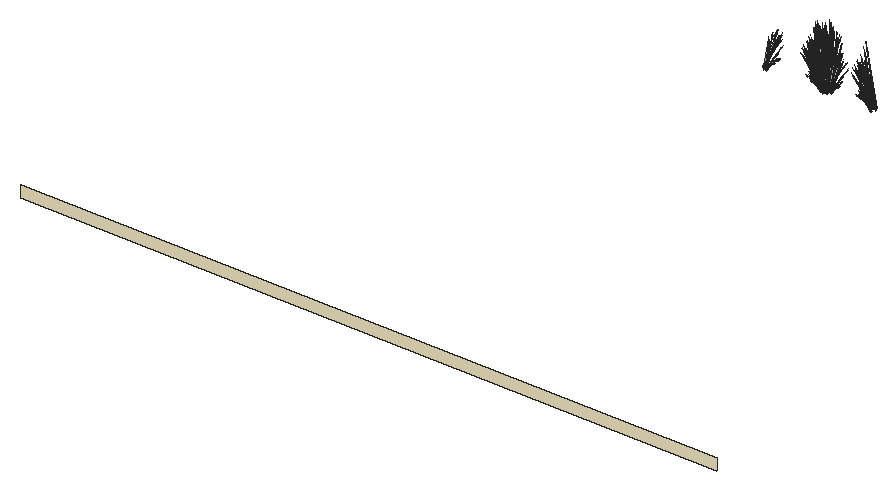
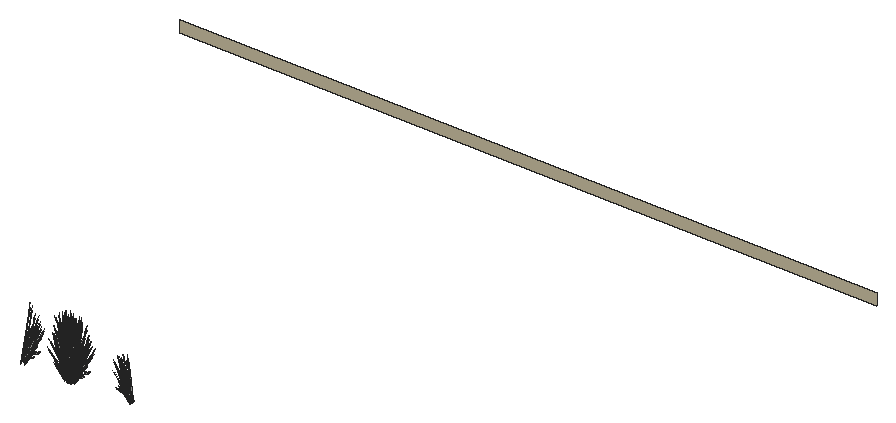
# SketchUp Ruby script. Lengths in inches.
U = 1.inch
M = Sketchup.active_model
def pt(a) = Geom::Point3d.new(a.map { |v| v * U })
def face(e, loops, mat)
  f = e.add_face(loops[0].map { |a| pt(a) })
  loops[1..].each { |l| e.add_face(l.map { |a| pt(a) }).erase! }
  f.material = f.back_material = mat if mat
  f
end
# faces: each face lists its corners as indices into pts; further lists are holes
def faces(e, pts, list, mat = nil) = list.each { |f| face(e, (f[0].is_a?(Array) ? f : [f]).map { |l| l.map { |i| pts[i] } }, mat) }
# xy, xz, yz: faces in a plane at the given z, y or x. An outline is a flat list of corners, or four numbers for a rectangle; further outlines are holes
def ring(l) = l.size == 4 ? [[l[0], l[1]], [l[2], l[1]], [l[2], l[3]], [l[0], l[3]]] : l.each_slice(2).to_a
def flat(e, list, mat, &to3) = list.each { |f| face(e, (f[0].is_a?(Array) ? f : [f]).map { |l| ring(l).map { |u, v| to3.(u, v) } }, mat) }
def xy(e, z, list, mat = nil) = flat(e, list, mat) { |x, y| [x, y, z] }
def xz(e, y, list, mat = nil) = flat(e, list, mat) { |x, z| [x, y, z] }
def yz(e, x, list, mat = nil) = flat(e, list, mat) { |y, z| [x, y, z] }
def lines(e, pts, list) = list.each { |a, b| e.add_line(pt(pts[a]), pt(pts[b])) }
# prism: a flat outline (further loops are holes) pulled along v
def prism(e, loops, v, mat = nil)
  f = face(e, loops, mat); d = Geom::Vector3d.new(v.map { |x| x * U })
  f.pushpull(f.normal.samedirection?(d) ? d.length : -d.length)
end
def box(e, o, s, mat = nil) = prism(e, [[o, [o[0] + s[0], o[1], o[2]], [o[0] + s[0], o[1] + s[1], o[2]], [o[0], o[1] + s[1], o[2]]]], [0, 0, s[2]], mat)
def at(x, y, z, deg = 0) = Geom::Transformation.translation(pt([x, y, z])) * Geom::Transformation.rotation(ORIGIN, Z_AXIS, deg.degrees)
def axes(o, x, y, z) = Geom::Transformation.new([*x, 0, *y, 0, *z, 0, *pt(o).to_a, 1])
def part(name) = M.definitions.add(name)
# library, detail: a bought-in or finely detailed component or shape, given as its bounding box
def library(name, o, s) = part(name).tap { |d| box(d.entities, o, s) }
def detail(e, o, s) = box(e.add_group.entities, o, s)
def put(e, d, t, mat = nil) = e.add_instance(d, t).tap { |i| i.material = mat if mat }
def group(e, t, mat = nil) = e.add_group.tap { |g| g.transformation = t; g.material = mat if mat }.entities
root = M.entities
M.materials.add("D01_Frost_White").color = [255, 242, 206]
M.materials.add("LightPink_Translucent").color = [144, 107, 117]
M.materials["LightPink_Translucent"].alpha = 0.75
c1 = part("blade")
p = [[2.15,0.21,22],[0,0.17,0],[0.09,0.45,0],[2.18,0.31,22],[2.29,0.31,22],[0.38,0.45,0],
  [2.48,0.24,33],[2.49,0.24,33],[2.48,0.22,33]]
faces(c1.entities,p,[[0,1,2,3],[4,5,2,3],[6,3,4,7],[8,0,3,6]])
c2 = part("seeds")
p = [[0.3,-0.1,1.38],[-0.01,-0.03,1.59],[-0.01,-0.03,0.03],[0.14,-0.07,-0.07],[0.29,-0.03,3],[0.15,0.01,3.11]]
faces(c2.entities,p,[[0,1,2,3],[1,0,4,5]],"LightPink_Translucent")
c3 = part("blade with seeds")
put(c3.entities,c1,at(0,0,0))
put(c3.entities,c2,axes([2.4,0.25,30.99],[1.5799,-0.05474,1.17369],[-0.12525,1.92788,0.29478],[-0.07173,-0.02425,1.56792]))
xz(root,18,[[492,-6,852,0]],"D01_Frost_White")
put(root,c3,axes([668.69,277.87,2.26],[0.40003,-0.04673,-0.17707],[0.10563,0.26712,0.2286],[0.11464,-0.07175,0.4374]))
put(root,c3,axes([668.375,277.96,2.49],[0.24005,-0.25798,-0.35523],[0.42065,0.18334,0.04287],[0.14333,-0.09347,0.5025]))
put(root,c3,axes([668.78,278.75,2.37],[0.16879,0.22293,0.03215],[-0.30779,0.10912,0.2531],[0.13568,-0.02153,0.38595]))
put(root,c3,axes([668.37,279.35,2.26],[0.26148,0.20471,-0.17707],[-0.29857,0.19378,0.2286],[0.1517,0.02948,0.4374]))
put(root,c3,axes([668.07,279.375,2.52],[0.02461,-0.33251,-0.0608],[0.4659,0.00909,-0.33747],[0.17944,0.0231,0.51278]))
put(root,c3,axes([668.59,278.76,2.52],[-0.23123,-0.29606,-0.0608],[0.41039,-0.14549,-0.33747],[0.17294,-0.03906,0.51278]))
put(root,c3,axes([668.75,278.67,2.37],[-0.12984,0.29812,0.24001],[-0.42685,-0.10194,0.1979],[0.16786,-0.01792,0.49665]))
put(root,c3,axes([668.48,279.17,2.36],[0.09858,-0.00553,0.87472],[0.2704,-0.25401,-0.13834],[0.17535,0.03353,0.07015]))
put(root,c3,axes([668.57,278.5,2.34],[0.1245,-0.29741,-0.25549],[0.42685,0.10194,-0.1979],[0.17186,-0.02727,0.48886]))
put(root,c3,axes([669.64,278.69,1.38],[-0.28394,0.05398,0.5743],[0.13365,-0.22308,0.42196],[0.15063,0.01526,0.12649]))
put(root,c3,axes([668.72,277.72,1.3],[-0.16417,-0.00968,0.71501],[-0.16819,-0.25979,-0.15377],[0.20169,-0.07349,0.3057]))
put(root,c3,axes([668.83,278.64,2.26],[0.38192,0.09121,-0.17707],[-0.11139,0.2661,0.2286],[0.15377,-0.0244,0.4374]))
put(root,c3,axes([668.1,279.21,2.49],[0.45939,0.00787,-0.35523],[-0.03085,0.3315,0.04287],[0.19462,0.03498,0.5025]))
put(root,c3,axes([669.03,278.59,0.99],[-0.29599,0.03924,0.70792],[-0.04711,-0.31232,0.04052],[0.20731,-0.04727,0.40283]))
put(root,c3,axes([669.35,278.38,0.75],[-0.02402,-0.04964,0.88171],[0.16658,-0.29036,-0.1347],[0.16804,-0.00418,0.15018]))
put(root,c3,axes([669.51,279.64,2.35],[-0.04155,-0.02862,0.88692],[0.0909,-0.30682,-0.08381],[0.16368,-0.0196,0.15695]))
put(root,c3,axes([667.79,278.31,1.9375],[-0.19062,0.00741,0.85688],[0.12645,-0.32094,0.06928],[0.27165,0.01985,0.36631]))
put(root,c3,axes([668.49,278.61,2.49],[0.40382,-0.1444,-0.35523],[0.22505,0.29724,0.04287],[0.19512,-0.03377,0.5025]))
put(root,c3,axes([669.85,278.29,2.36],[0.06377,-0.0498,0.87472],[-0.08162,-0.30549,-0.13834],[0.16001,-0.05792,0.07015]))
put(root,c3,axes([669.11,279.05,1.3],[-0.11068,-0.08041,0.71501],[0.144,-0.26601,-0.15377],[0.22393,0.03604,0.3057]))
put(root,c3,axes([697.02,279.34,1.9375],[0.19062,-0.00741,0.85688],[-0.12645,0.32094,0.06928],[-0.27165,-0.01985,0.36631]))
put(root,c3,axes([698.02,279.57,1.67],[0.13063,-0.0473,0.88532],[0.04505,0.33024,0.06928],[-0.28294,0.04382,0.31642]))
put(root,c3,axes([696.61,279.79,2.36],[-0.07505,0.04245,0.87472],[0.00638,0.31015,-0.13834],[-0.17202,0.04033,0.07015]))
put(root,c3,axes([697.59,279.04,2.49],[-0.45939,-0.00787,-0.35523],[0.03085,-0.3315,0.04287],[-0.19462,-0.03498,0.5025]))
put(root,c3,axes([697.22,279.125,1.3],[0.08973,0.09103,0.71501],[-0.20675,0.24743,-0.15377],[-0.2123,-0.05914,0.3057]))
put(root,c3,axes([696.86,279.62,2.26],[-0.38192,-0.09121,-0.17707],[0.11139,-0.2661,0.2286],[-0.15377,0.0244,0.4374]))
put(root,c3,axes([697.38,278.83,1.9375],[0.1707,0.05633,0.85688],[-0.35326,0.23632,0.06928],[-0.22018,-0.10661,0.36631]))
put(root,c3,axes([697.12,279.75,2.34],[-0.1245,0.29741,-0.25549],[-0.42685,-0.10194,-0.1979],[-0.17186,0.02727,0.48886]))
put(root,c3,axes([697.44,279.11,2.34],[-0.3337,0.21658,-0.25549],[-0.29224,-0.22879,-0.1979],[-0.16955,-0.03295,0.48886]))
put(root,c3,axes([696.9,279.73,0.75],[0.01165,0.05153,0.88171],[-0.23495,0.26909,-0.1347],[-0.16689,-0.01356,0.15018]))
put(root,c3,axes([696.97,278.5,2.35],[0.03407,0.03263,0.88692],[-0.16424,0.29331,-0.08381],[-0.16634,0.00212,0.15695]))
put(root,c3,axes([697.35,278.31,2.36],[-0.09888,-0.00231,0.87472],[-0.3148,0.23079,-0.13834],[-0.16797,-0.04716,0.07015]))
put(root,c3,axes([696.94,279.58,2.37],[0.12984,-0.29812,0.24001],[0.42685,0.10194,0.1979],[-0.16786,0.01792,0.49665]))
put(root,c3,axes([697.1,279.5,2.52],[0.23123,0.29606,-0.0608],[-0.41039,0.14549,-0.33747],[-0.17294,0.03906,0.51278]))
put(root,c3,axes([697.62,278.88,2.52],[-0.02461,0.33251,-0.0608],[-0.4659,-0.00909,-0.33747],[-0.17944,-0.0231,0.51278]))
put(root,c3,axes([697.32,278.91,2.26],[-0.26148,-0.20471,-0.17707],[0.29857,-0.19378,0.2286],[-0.1517,-0.02948,0.4374]))
put(root,c3,axes([696.91,279.5,2.37],[-0.16879,-0.22293,0.03215],[0.30779,-0.10912,0.2531],[-0.13568,0.02153,0.38595]))
put(root,c3,axes([696.6875,279.4,1.38],[0.2934,-0.0234,0.5743],[-0.18611,0.20614,0.42196],[-0.14499,-0.03092,0.12649]))
put(root,c3,axes([697.28,278.83,2.55],[0.37952,-0.24129,0.26881],[0.32731,0.25625,0.22165],[-0.17806,-0.04451,0.55625]))
put(root,c3,axes([697.26,279.59,2.53],[0.38192,0.09121,0.17707],[-0.11139,0.2661,-0.2286],[-0.15377,0.0244,0.4374]))
put(root,c3,axes([697.45,278.83,2.37],[0.02314,-0.24862,0.03215],[0.34943,0.00682,0.2531],[-0.13385,-0.02602,0.38595]))
put(root,c3,axes([698.4375,280.2,1.03],[-0.47805,-0.0536,-0.31177],[0.10088,-0.33065,-0.08182],[-0.14266,-0.04007,0.68817]))
put(root,c3,axes([698.53,278.4,2.72],[-0.30671,0.31344,-0.0681],[-0.44417,-0.18058,-0.37797],[-0.1544,-0.08856,0.57432]))
put(root,c3,axes([697.6875,279.01,2.53],[0.26148,0.20471,0.17707],[-0.29857,0.19378,-0.2286],[-0.1517,-0.02948,0.4374]))
put(root,c3,axes([698.39,278.65,2.49],[-0.39186,-0.15803,-0.35523],[0.27849,-0.27693,0.04287],[-0.14198,-0.09436,0.5025]))
put(root,c3,axes([698.21,278.66,2.34],[-0.45348,0.07772,-0.25549],[-0.07933,-0.29434,-0.1979],[-0.1218,-0.08435,0.48886]))
put(root,c3,axes([697.8125,280.83,1.01],[-0.4301,-0.16348,-0.24825],[0.25708,-0.29314,0],[-0.09796,-0.03723,0.78752]))
put(root,c3,axes([697.625,278.39,0.75],[-0.04451,0.04307,0.88171],[-0.44986,0.09286,-0.1347],[-0.10868,-0.08448,0.15018]))
put(root,c3,axes([698.07,281.02,1.1875],[-0.28732,0.32763,0],[-0.4807,-0.18271,-0.25804],[-0.10948,-0.04161,0.81856]))
put(root,c3,axes([697.34,278.56,1.0625],[-0.13257,0.26698,-0.01946],[-0.40802,-0.08212,-0.08825],[-0.06195,-0.04367,0.29107]))
put(root,c3,axes([698.41,277.65,2.35],[-0.00857,0.03919,0.88692],[-0.42284,0.14223,-0.08381],[-0.12443,-0.0727,0.15695]))
put(root,c3,axes([697.95,278.22,1.3],[-0.02783,0.10696,0.71501],[-0.40683,0.08954,-0.15377],[-0.0951,-0.13825,0.3057]))
put(root,c3,axes([698.09,278.5,1.9375],[0.10505,0.10498,0.85688],[-0.48542,0.08838,0.06928],[-0.10971,-0.1648,0.36631]))
put(root,c3,axes([698.98,280.25,1.33],[-0.46399,0.21707,-0.14548],[-0.30855,-0.30672,-0.25001],[-0.11448,-0.03115,0.79854]))
put(root,c3,axes([698.26,278.44,2.26],[-0.07098,-0.26335,-0.17707],[0.40574,-0.06954,0.2286],[-0.10898,-0.07547,0.4374]))
put(root,c3,axes([697.125,279.78,1.1875],[-0.57465,0,0],[0,-0.36542,-0.25804],[0,-0.08323,0.81856]))
put(root,c3,axes([697.93,280.7,1.01],[-0.10795,-0.28489,-0.15489],[0.42874,-0.0809,0.15489],[-0.08643,-0.03285,0.69487]))
put(root,c3,axes([698.5,278.66,2.53],[0.07098,0.26335,0.17707],[-0.40574,0.06954,-0.2286],[-0.10898,-0.07547,0.4374]))
put(root,c3,axes([697.57,279.68,1.17],[-0.42746,0.27488,0.15378],[-0.42772,-0.27199,-0.18246],[-0.01493,-0.07806,0.82443]))
put(root,c3,axes([699.33,280.44,1.66],[0.39713,0.13184,0.7563],[-0.38905,0.28403,0.29908],[-0.17427,-0.16834,0.63403]))
put(root,c3,axes([697.8125,278.05,1.38],[0.23972,0.1138,0.5743],[-0.34912,0.06841,0.42196],[-0.0747,-0.08746,0.12649]))
put(root,c3,axes([699.5,280.35,1.23],[-0.44875,-0.26316,-0.12596],[0.3776,-0.2955,0.27565],[-0.12084,0.03078,0.84108]))
put(root,c3,axes([698.6875,280.1,1.11],[-0.27607,-0.27443,-0.2237],[0.41817,-0.19325,0.10766],[-0.08934,-0.03396,0.71822]))
put(root,c3,axes([698.3125,278.35,2.55],[0.51193,-0.08404,0.26881],[0.08885,0.32966,0.22165],[-0.1204,-0.09716,0.55625]))
put(root,c3,axes([699.28,280.29,1.11],[-0.49904,0.02018,-0.2237],[-0.04513,-0.33504,0.10766],[-0.08934,0.03396,0.71822]))
put(root,c3,axes([698.43,278.42,2.37],[0.20887,-0.2077,0.03215],[0.29744,0.12092,0.2531],[-0.09616,-0.06659,0.38595]))
put(root,c3,axes([698.32,280.85,1.24],[0.4301,0.16348,0.24825],[-0.25708,0.29314,0],[-0.09796,-0.03723,0.78752]))
put(root,c3,axes([698.73,280.25,1.22],[0.1218,-0.38743,-0.11714],[0.57753,0.06753,0.25635],[-0.10091,-0.0535,0.7822]))
put(root,c3,axes([698.9375,280.34,1.31],[-0.08866,0.29179,0.0724],[-0.43315,-0.05065,-0.20674],[-0.07883,-0.02996,0.63372]))
put(root,c3,axes([698.89,277.8,2.36],[-0.07029,-0.04584,0.87472],[-0.46908,0.02906,-0.13834],[-0.07486,-0.10965,0.07015]))
put(root,c3,axes([697.25,279.53,1.01],[0,-0.32696,-0.24825],[0.51416,0,0],[0,-0.07447,0.78752]))
put(root,c3,axes([697.47,279.83,1.24],[0,0.32696,0.24825],[-0.51416,0,0],[0,-0.07447,0.78752]))
put(root,c3,axes([698.6,279.91,1.33],[-0.51755,-0.15601,-0.14548],[0.2492,-0.32927,-0.25001],[-0.01626,-0.08084,0.79854]))
put(root,c3,axes([698.37,279.57,1.05],[-0.18873,-0.33528,-0.34918],[0.54365,-0.12075,-0.09164],[-0.02086,-0.11353,0.77075]))
put(root,c3,axes([699.6,278.51,2.52],[-0.44971,0.15222,-0.0608],[-0.221,-0.27017,-0.33747],[-0.05933,-0.11385,0.51278]))
put(root,c3,axes([699.22,278.52,2.34],[-0.45175,-0.08196,-0.25549],[0.15485,-0.28101,-0.1979],[-0.04142,-0.11314,0.48886]))
put(root,c3,axes([697.47,279.54,1.01],[0.32079,-0.20399,-0.15489],[0.32079,0.20399,0.15489],[0,-0.06571,0.69487]))
put(root,c3,axes([698.92,278.22,1.0625],[-0.31757,0.18757,-0.01946],[-0.29098,-0.20543,-0.08825],[-0.02049,-0.05821,0.29107]))
put(root,c3,axes([698.79,280.07,1.18],[0.58084,0.06889,0.22877],[-0.11821,0.38906,0.08977],[-0.08488,-0.03757,0.79428]))
put(root,c3,axes([698.64,280,1.36],[-0.22297,0.29461,0.2237],[-0.4633,-0.14179,-0.10766],[0,-0.06791,0.71822]))
put(root,c3,axes([699.38,278.58,2.49],[-0.21934,-0.26585,-0.35523],[0.45151,-0.14816,0.04287],[-0.05129,-0.12845,0.5025]))
put(root,c3,axes([698.48,280.6875,1.24],[0.49383,-0.08678,0.08821],[0.12194,0.32295,0.17543],[-0.04404,-0.04705,0.80203]))
put(root,c3,axes([699.12,280.74,1.1],[-0.4633,-0.14679,0],[0.22297,-0.30501,0],[0,0,0.81353]))
put(root,c3,axes([699.47,278.62,2.53],[-0.13855,0.25143,0.17707],[-0.4042,-0.07334,-0.2286],[-0.03706,-0.10123,0.4374]))
put(root,c3,axes([699.95,280.71,1.24],[0.13276,-0.32494,0.08821],[0.4858,0.09195,0.17543],[-0.08392,0.00158,0.80203]))
put(root,c3,axes([699.61,280.03,1.15],[-0.42746,-0.28142,-0.03066],[0.42772,-0.28159,0],[-0.01493,-0.00983,0.87786]))
put(root,c3,axes([699.72,280.13,1.36],[0.49904,-0.02018,0.2237],[0.04513,0.33504,-0.10766],[-0.08934,0.03396,0.71822]))
put(root,c3,axes([699,277.99,0.75],[-0.07708,0.01178,0.88171],[-0.42627,-0.1326,-0.1347],[0.00715,-0.1106,0.15018]))
put(root,c3,axes([699.42,278.35,2.26],[0.13855,-0.25143,-0.17707],[0.4042,0.07334,0.2286],[-0.03706,-0.10123,0.4374]))
put(root,c3,axes([698.74,279.71,1.18],[0.1998,0.3656,0.22877],[-0.5709,0.12713,0.08977],[0.00698,-0.06718,0.79428]))
put(root,c3,axes([698.65,279.66,1.11],[0.22297,-0.29461,-0.2237],[0.4633,0.14179,0.10766],[0,-0.06791,0.71822]))
put(root,c3,axes([699.22,280.61,1.1],[-0.14994,-0.28188,0],[0.42817,-0.09871,0],[0,0,0.77185]))
put(root,c3,axes([699.59,278.39,2.37],[0.33863,-0.11112,0.03215],[0.16575,0.20263,0.2531],[-0.0327,-0.08932,0.38595]))
put(root,c3,axes([700.71,279.875,1.24],[-0.36107,-0.23816,0.08821],[0.36387,-0.231,0.17543],[-0.03988,0.04864,0.80203]))
put(root,c3,axes([699.46,279.74,1.1],[0,-0.37831,0],[0.57465,0,0],[0,0,0.89728]))
put(root,c3,axes([699.47,278.41,2.37],[0.45283,0.08548,0.24001],[-0.15485,0.28101,0.1979],[-0.02721,-0.11051,0.49665]))
put(root,c3,axes([698.93,279.81,1.22],[0.5178,0.15847,0.12032],[-0.2492,0.32927,0.25001],[0,-0.0759,0.80271]))
put(root,c3,axes([699.75,279.89,1.15],[0,0.37813,-0.02818],[-0.57465,0,0],[0,0.01188,0.89684]))
put(root,c3,axes([698.76,279.59,1.36],[-0.49904,0.02018,0.2237],[-0.04513,-0.33504,-0.10766],[0.08934,-0.03396,0.71822]))
put(root,c3,axes([698.53,279.01,1.24],[-0.13276,0.32494,0.08821],[-0.4858,-0.09195,0.17543],[0.08392,-0.00158,0.80203]))
put(root,c3,axes([698.29,278.61,1.1875],[-0.28732,-0.32763,0],[0.4807,-0.18271,-0.25804],[0.10948,-0.04161,0.81856]))
put(root,c3,axes([700,279.03,1.24],[-0.49383,0.08678,0.08821],[-0.12194,-0.32295,0.17543],[0.04404,0.04705,0.80203]))
put(root,c3,axes([699.49,277.82,1.38],[0.05895,0.19066,0.5743],[-0.32704,-0.1056,0.42196],[0.03519,-0.09762,0.12649]))
put(root,c3,axes([699.19,279.5,1.18],[-0.38104,0.29672,0.22877],[-0.45269,-0.26192,0.08977],[0.09186,-0.02961,0.79428]))
put(root,c3,axes([699.84,279.97,1.11],[0.32079,0.21119,0],[-0.32079,0.21119,0],[0,0,0.84633]))
put(root,c3,axes([699.84,279.72,1.36],[0.22297,-0.29461,0.2237],[0.4633,0.14179,-0.10766],[0,0.06791,0.71822]))
put(root,c3,axes([699.64,280.74,1.1],[0.4633,0.14679,0],[-0.22297,0.30501,0],[0,0,0.87477]))
put(root,c3,axes([699.6875,279.65,1.19],[-0.58084,-0.06889,0.24599],[0.11821,-0.38906,0.09653],[0.08488,0.03757,0.85407]))
put(root,c3,axes([700.9,278.13,2.35],[-0.04667,0.02497,0.88692],[-0.45726,-0.08426,-0.08381],[-0.01655,-0.10898,0.15695]))
put(root,c3,axes([700.54,278.85,2.52],[-0.50507,-0.0162,-0.0608],[0.01381,-0.30672,-0.33747],[0.03508,-0.11813,0.51278]))
put(root,c3,axes([699.85,279.82,1.1],[0.51416,0,0],[0,0.33849,0],[0,0,0.89203]))
put(root,c3,axes([700.34,278.9,2.53],[-0.31095,0.17214,0.17707],[-0.29435,-0.19656,-0.2286],[0.04479,-0.09987,0.4374]))
put(root,c3,axes([699.36,279.45,1.36],[-0.27607,-0.27443,0.2237],[0.41817,-0.19325,-0.10766],[0.08934,0.03396,0.71822]))
put(root,c3,axes([698.86,279.52,1.33],[-0.05355,-0.37308,-0.14548],[0.55775,-0.02256,-0.25001],[0.09822,-0.04969,0.79854]))
put(root,c3,axes([700.03,279.79,1.31],[0.42817,-0.09535,0.0724],[0.14994,0.27228,-0.20674],[0,0.05992,0.63372]))
put(root,c3,axes([700.19,278.74,2.34],[-0.32898,-0.21969,-0.25549],[0.34753,-0.1924,-0.1979],[0.05006,-0.11162,0.48886]))
put(root,c3,axes([698.78,278.69,1.01],[0.42874,0.0809,-0.15489],[-0.10795,0.28489,0.15489],[0.08643,-0.03285,0.69487]))
put(root,c3,axes([699.98,278.35,1.3],[-0.13063,0.06618,0.71501],[-0.39122,-0.11583,-0.15377],[0.07252,-0.14406,0.3057]))
put(root,c3,axes([701.01,279.89,1.24],[0,-0.32696,0.24825],[0.51416,0,0],[0,0.07447,0.78752]))
put(root,c3,axes([698.68,278.56,1.01],[0.4301,-0.16348,-0.24825],[0.25708,0.29314,0],[0.09796,-0.03723,0.78752]))
put(root,c3,axes([699.54,279.375,1.31],[0.08866,-0.29179,0.0724],[0.43315,0.05065,-0.20674],[0.07883,0.02996,0.63372]))
put(root,c3,axes([700.16,278.86,1.24],[-0.4301,-0.16348,0.24825],[0.25708,-0.29314,0],[0.09796,0.03723,0.78752]))
put(root,c3,axes([700.29,278.84,2.49],[0.01196,-0.30243,-0.35523],[0.50354,0.02031,0.04287],[0.05314,-0.12813,0.5025]))
put(root,c3,axes([699.78,280.57,1.09],[0.48247,-0.11094,-0.09599],[0.16954,0.31956,0.00004],[0.05326,-0.01226,0.86949]))
put(root,c3,axes([699.79,279.62,1.11],[0.27607,0.27443,-0.2237],[-0.41817,0.19325,0.10766],[0.08934,0.03396,0.71822]))
put(root,c3,axes([700.5,278.65,2.26],[0.31095,-0.17214,-0.17707],[0.29435,0.19656,0.2286],[0.04479,-0.09987,0.4374]))
put(root,c3,axes([700.62,278.74,2.37],[0.37765,0.01523,0.03215],[-0.01035,0.23004,0.2531],[0.03952,-0.08812,0.38595]))
put(root,c3,axes([701,278.36,2.36],[-0.00444,-0.06507,0.87472],[-0.37468,-0.18807,-0.13834],[0.05793,-0.114,0.07015]))
put(root,c3,axes([699.19,279.23,1.03],[0.30954,-0.24575,-0.31177],[0.38452,0.22284,-0.08182],[0.12404,-0.0613,0.68817]))
put(root,c3,axes([700.5,278.72,2.37],[0.32725,0.22308,0.24001],[-0.34753,0.1924,0.1979],[0.06036,-0.10466,0.49665]))
put(root,c3,axes([700.55,279.01,1.01],[0.10795,0.28489,-0.15489],[-0.42874,0.0809,0.15489],[0.08643,0.03285,0.69487]))
put(root,c3,axes([699.5,279.47,1.33],[0.46399,-0.21707,-0.14548],[0.30855,0.30672,-0.25001],[0.11448,0.03115,0.79854]))
put(root,c3,axes([700.88,279.43,2.53],[-0.40003,0.04673,0.17707],[-0.10563,-0.26712,-0.2286],[0.11464,-0.07175,0.4374]))
put(root,c3,axes([699.73,278.68,1.9375],[-0.08557,0.11238,0.85688],[-0.35897,-0.23257,0.06928],[0.16194,-0.14495,0.36631]))
put(root,c3,axes([698.33,279.27,0.8],[-0.45234,0.1309,0.64464],[-0.14398,-0.37559,0.25048],[0.27777,0.00625,0.73321]))
put(root,c3,axes([701.09,279.46,2.52],[-0.4251,-0.18028,-0.0608],[0.24491,-0.26108,-0.33747],[0.1201,-0.09075,0.51278]))
put(root,c3,axes([700.41,278.69,1.1875],[0.28732,-0.32763,0],[0.4807,0.18271,-0.25804],[0.10948,0.04161,0.81856]))
put(root,c3,axes([700.89,278.55,0.75],[-0.06878,-0.02576,0.88171],[-0.17668,-0.28776,-0.1347],[0.11919,-0.07809,0.15018]))
put(root,c3,axes([700.51,280.64,2.53],[-0.26148,-0.20471,0.17707],[0.29857,-0.19378,-0.2286],[0.1517,0.02948,0.4374]))
put(root,c3,axes([700.67,278.89,1.01],[0.4301,0.16348,-0.24825],[-0.25708,0.29314,0],[0.09796,0.03723,0.78752]))
put(root,c3,axes([700.875,279.24,2.34],[-0.11806,-0.29854,-0.25549],[0.44709,-0.05222,-0.1979],[0.12812,-0.08019,0.48886]))
put(root,c3,axes([701.66,280.78,1.96],[-0.08796,-0.27485,-0.01746],[0.41573,-0.06319,-0.07916],[0.08682,0.01742,0.26109]))
put(root,c3,axes([700.94,280.07,2.53],[-0.38192,-0.09121,0.17707],[0.11139,-0.2661,-0.2286],[0.15377,-0.0244,0.4374]))
put(root,c3,axes([700.04,279.52,1.03],[0.47805,0.0536,-0.31177],[-0.10088,0.33065,-0.08182],[0.14266,0.04007,0.68817]))
put(root,c3,axes([702.08,279.71,1.13],[-0.28491,-0.20907,-0.03244],[0.31204,-0.19157,-0.14708],[0.08842,-0.01349,0.48512]))
put(root,c3,axes([701.42,278.65,1.38],[-0.15307,0.16644,0.5743],[-0.13157,-0.22361,0.42196],[0.12643,-0.05603,0.12649]))
put(root,c3,axes([701.24,279.39,2.37],[0.31549,0.13751,0.03215],[-0.18368,0.19581,0.2531],[0.10115,-0.06331,0.38595]))
put(root,c3,axes([701.15,279.33,2.37],[0.11397,0.30091,0.24001],[-0.44709,0.05222,0.1979],[0.13177,-0.07077,0.49665]))
put(root,c3,axes([702.13,279.38,2.35],[-0.06002,-0.00248,0.88692],[-0.24926,-0.26607,-0.08381],[0.1001,-0.08748,0.15695]))
put(root,c3,axes([701.2,279.27,2.26],[0.40003,-0.04673,-0.17707],[0.10563,0.26712,0.2286],[0.11464,-0.07175,0.4374]))
put(root,c3,axes([700.89,279.36,2.49],[0.24005,-0.25798,-0.35523],[0.42065,0.18334,0.04287],[0.14333,-0.09347,0.5025]))
put(root,c3,axes([701.29,280.15,2.37],[0.16879,0.22293,0.03215],[-0.30779,0.10912,0.2531],[0.13568,-0.02153,0.38595]))
put(root,c3,axes([700.58,280.77,2.52],[0.02461,-0.33251,-0.0608],[0.4659,0.00909,-0.33747],[0.17944,0.0231,0.51278]))
put(root,c3,axes([701.1,280.16,2.52],[-0.23123,-0.29606,-0.0608],[0.41039,-0.14549,-0.33747],[0.17294,-0.03906,0.51278]))
put(root,c3,axes([701.26,280.07,2.37],[-0.12984,0.29812,0.24001],[-0.42685,-0.10194,0.1979],[0.16786,-0.01792,0.49665]))
put(root,c3,axes([701.08,279.9,2.34],[0.1245,-0.29741,-0.25549],[0.42685,0.10194,-0.1979],[0.17186,-0.02727,0.48886]))
put(root,c3,axes([702.15,280.09,1.38],[-0.28394,0.05398,0.5743],[0.13365,-0.22308,0.42196],[0.15063,0.01526,0.12649]))
put(root,c3,axes([701.23,279.125,1.3],[-0.16417,-0.00968,0.71501],[-0.16819,-0.25979,-0.15377],[0.20169,-0.07349,0.3057]))
put(root,c3,axes([701.34,280.04,2.26],[0.38192,0.09121,-0.17707],[-0.11139,0.2661,0.2286],[0.15377,-0.0244,0.4374]))
put(root,c3,axes([701.54,279.99,0.99],[-0.29599,0.03924,0.70792],[-0.04711,-0.31232,0.04052],[0.20731,-0.04727,0.40283]))
put(root,c3,axes([701.86,279.78,0.75],[-0.02402,-0.04964,0.88171],[0.16658,-0.29036,-0.1347],[0.16804,-0.00418,0.15018]))
put(root,c3,axes([702.02,281.04,2.35],[-0.04155,-0.02862,0.88692],[0.0909,-0.30682,-0.08381],[0.16368,-0.0196,0.15695]))
put(root,c3,axes([700.3,279.71,1.9375],[-0.19062,0.00741,0.85688],[0.12645,-0.32094,0.06928],[0.27165,0.01985,0.36631]))
put(root,c3,axes([701,280.01,2.49],[0.40382,-0.1444,-0.35523],[0.22505,0.29724,0.04287],[0.19512,-0.03377,0.5025]))
put(root,c3,axes([702.36,279.69,2.36],[0.06377,-0.0498,0.87472],[-0.08162,-0.30549,-0.13834],[0.16001,-0.05792,0.07015]))
put(root,c3,axes([701.62,280.45,1.3],[-0.11068,-0.08041,0.71501],[0.144,-0.26601,-0.15377],[0.22393,0.03604,0.3057]))
put(root,c3,axes([723.13,279.29,1.9375],[0.19062,-0.00741,0.85688],[-0.12645,0.32094,0.06928],[-0.27165,-0.01985,0.36631]))
put(root,c3,axes([724.125,279.52,1.67],[0.13063,-0.0473,0.88532],[0.04505,0.33024,0.06928],[-0.28294,0.04382,0.31642]))
put(root,c3,axes([722.72,279.74,2.36],[-0.07505,0.04245,0.87472],[0.00638,0.31015,-0.13834],[-0.17202,0.04033,0.07015]))
put(root,c3,axes([723.7,278.99,2.49],[-0.45939,-0.00787,-0.35523],[0.03085,-0.3315,0.04287],[-0.19462,-0.03498,0.5025]))
put(root,c3,axes([723.33,279.07,1.3],[0.08973,0.09103,0.71501],[-0.20675,0.24743,-0.15377],[-0.2123,-0.05914,0.3057]))
put(root,c3,axes([722.96,279.57,2.26],[-0.38192,-0.09121,-0.17707],[0.11139,-0.2661,0.2286],[-0.15377,0.0244,0.4374]))
put(root,c3,axes([723.49,278.78,1.9375],[0.1707,0.05633,0.85688],[-0.35326,0.23632,0.06928],[-0.22018,-0.10661,0.36631]))
put(root,c3,axes([723.23,279.7,2.34],[-0.1245,0.29741,-0.25549],[-0.42685,-0.10194,-0.1979],[-0.17186,0.02727,0.48886]))
put(root,c3,axes([723.55,279.06,2.34],[-0.3337,0.21658,-0.25549],[-0.29224,-0.22879,-0.1979],[-0.16955,-0.03295,0.48886]))
put(root,c3,axes([723.01,279.68,0.75],[0.01165,0.05153,0.88171],[-0.23495,0.26909,-0.1347],[-0.16689,-0.01356,0.15018]))
put(root,c3,axes([723.08,278.45,2.35],[0.03407,0.03263,0.88692],[-0.16424,0.29331,-0.08381],[-0.16634,0.00212,0.15695]))
put(root,c3,axes([723.46,278.26,2.36],[-0.09888,-0.00231,0.87472],[-0.3148,0.23079,-0.13834],[-0.16797,-0.04716,0.07015]))
put(root,c3,axes([723.05,279.53,2.37],[0.12984,-0.29812,0.24001],[0.42685,0.10194,0.1979],[-0.16786,0.01792,0.49665]))
put(root,c3,axes([723.2,279.45,2.52],[0.23123,0.29606,-0.0608],[-0.41039,0.14549,-0.33747],[-0.17294,0.03906,0.51278]))
put(root,c3,axes([723.72,278.83,2.52],[-0.02461,0.33251,-0.0608],[-0.4659,-0.00909,-0.33747],[-0.17944,-0.0231,0.51278]))
put(root,c3,axes([723.42,278.86,2.26],[-0.26148,-0.20471,-0.17707],[0.29857,-0.19378,0.2286],[-0.1517,-0.02948,0.4374]))
put(root,c3,axes([723.02,279.46,2.37],[-0.16879,-0.22293,0.03215],[0.30779,-0.10912,0.2531],[-0.13568,0.02153,0.38595]))
put(root,c3,axes([722.8,279.35,1.38],[0.2934,-0.0234,0.5743],[-0.18611,0.20614,0.42196],[-0.14499,-0.03092,0.12649]))
put(root,c3,axes([723.39,278.78,2.55],[0.37952,-0.24129,0.26881],[0.32731,0.25625,0.22165],[-0.17806,-0.04451,0.55625]))
put(root,c3,axes([723.37,279.54,2.53],[0.38192,0.09121,0.17707],[-0.11139,0.2661,-0.2286],[-0.15377,0.0244,0.4374]))
put(root,c3,axes([723.56,278.78,2.37],[0.02314,-0.24862,0.03215],[0.34943,0.00682,0.2531],[-0.13385,-0.02602,0.38595]))
put(root,c3,axes([724.55,280.15,1.03],[-0.47805,-0.0536,-0.31177],[0.10088,-0.33065,-0.08182],[-0.14266,-0.04007,0.68817]))
put(root,c3,axes([724.63,278.35,2.72],[-0.30671,0.31344,-0.0681],[-0.44417,-0.18058,-0.37797],[-0.1544,-0.08856,0.57432]))
put(root,c3,axes([723.8,278.96,2.53],[0.26148,0.20471,0.17707],[-0.29857,0.19378,-0.2286],[-0.1517,-0.02948,0.4374]))
put(root,c3,axes([724.5,278.6,2.49],[-0.39186,-0.15803,-0.35523],[0.27849,-0.27693,0.04287],[-0.14198,-0.09436,0.5025]))
put(root,c3,axes([724.32,278.61,2.34],[-0.45348,0.07772,-0.25549],[-0.07933,-0.29434,-0.1979],[-0.1218,-0.08435,0.48886]))
put(root,c3,axes([723.92,280.78,1.01],[-0.4301,-0.16348,-0.24825],[0.25708,-0.29314,0],[-0.09796,-0.03723,0.78752]))
put(root,c3,axes([723.73,278.34,0.75],[-0.04451,0.04307,0.88171],[-0.44986,0.09286,-0.1347],[-0.10868,-0.08448,0.15018]))
put(root,c3,axes([724.18,280.97,1.1875],[-0.28732,0.32763,0],[-0.4807,-0.18271,-0.25804],[-0.10948,-0.04161,0.81856]))
put(root,c3,axes([723.45,278.51,1.0625],[-0.13257,0.26698,-0.01946],[-0.40802,-0.08212,-0.08825],[-0.06195,-0.04367,0.29107]))
put(root,c3,axes([724.51,277.6,2.35],[-0.00857,0.03919,0.88692],[-0.42284,0.14223,-0.08381],[-0.12443,-0.0727,0.15695]))
